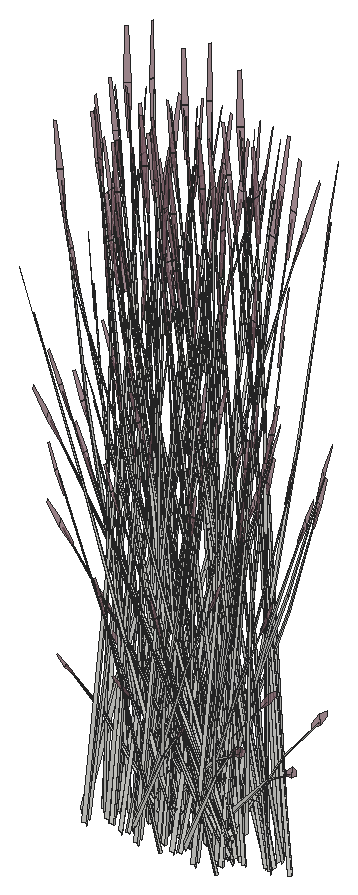
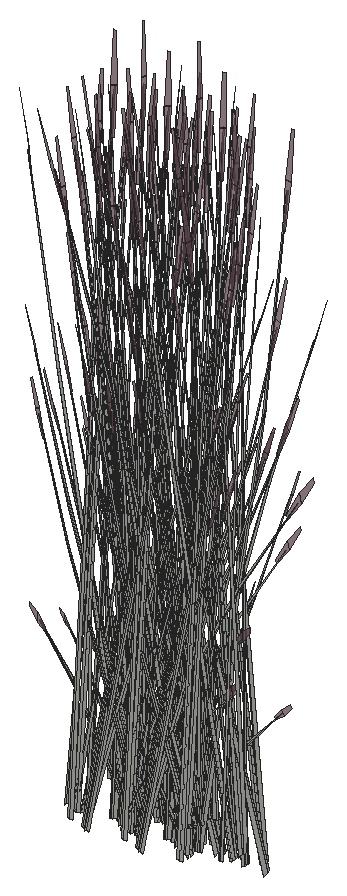
# SketchUp Ruby script. Lengths in inches.
U = 1.inch
M = Sketchup.active_model
def pt(a) = Geom::Point3d.new(a.map { |v| v * U })
def face(e, loops, mat)
  f = e.add_face(loops[0].map { |a| pt(a) })
  loops[1..].each { |l| e.add_face(l.map { |a| pt(a) }).erase! }
  f.material = f.back_material = mat if mat
  f
end
# faces: each face lists its corners as indices into pts; further lists are holes
def faces(e, pts, list, mat = nil) = list.each { |f| face(e, (f[0].is_a?(Array) ? f : [f]).map { |l| l.map { |i| pts[i] } }, mat) }
# xy, xz, yz: faces in a plane at the given z, y or x. An outline is a flat list of corners, or four numbers for a rectangle; further outlines are holes
def ring(l) = l.size == 4 ? [[l[0], l[1]], [l[2], l[1]], [l[2], l[3]], [l[0], l[3]]] : l.each_slice(2).to_a
def flat(e, list, mat, &to3) = list.each { |f| face(e, (f[0].is_a?(Array) ? f : [f]).map { |l| ring(l).map { |u, v| to3.(u, v) } }, mat) }
def xy(e, z, list, mat = nil) = flat(e, list, mat) { |x, y| [x, y, z] }
def xz(e, y, list, mat = nil) = flat(e, list, mat) { |x, z| [x, y, z] }
def yz(e, x, list, mat = nil) = flat(e, list, mat) { |y, z| [x, y, z] }
def lines(e, pts, list) = list.each { |a, b| e.add_line(pt(pts[a]), pt(pts[b])) }
# prism: a flat outline (further loops are holes) pulled along v
def prism(e, loops, v, mat = nil)
  f = face(e, loops, mat); d = Geom::Vector3d.new(v.map { |x| x * U })
  f.pushpull(f.normal.samedirection?(d) ? d.length : -d.length)
end
def box(e, o, s, mat = nil) = prism(e, [[o, [o[0] + s[0], o[1], o[2]], [o[0] + s[0], o[1] + s[1], o[2]], [o[0], o[1] + s[1], o[2]]]], [0, 0, s[2]], mat)
def at(x, y, z, deg = 0) = Geom::Transformation.translation(pt([x, y, z])) * Geom::Transformation.rotation(ORIGIN, Z_AXIS, deg.degrees)
def axes(o, x, y, z) = Geom::Transformation.new([*x, 0, *y, 0, *z, 0, *pt(o).to_a, 1])
def part(name) = M.definitions.add(name)
# library, detail: a bought-in or finely detailed component or shape, given as its bounding box
def library(name, o, s) = part(name).tap { |d| box(d.entities, o, s) }
def detail(e, o, s) = box(e.add_group.entities, o, s)
def put(e, d, t, mat = nil) = e.add_instance(d, t).tap { |i| i.material = mat if mat }
def group(e, t, mat = nil) = e.add_group.tap { |g| g.transformation = t; g.material = mat if mat }.entities
root = M.entities
M.materials.add("LightPink_Translucent").color = [144, 107, 117]
M.materials["LightPink_Translucent"].alpha = 0.75
c1 = part("blade")
p = [[2.15,0.21,22],[0,0.17,0],[0.09,0.45,0],[2.18,0.31,22],[2.29,0.31,22],[0.38,0.45,0],
  [2.48,0.24,33],[2.49,0.24,33],[2.48,0.22,33]]
faces(c1.entities,p,[[0,1,2,3],[4,5,2,3],[6,3,4,7],[8,0,3,6]])
c2 = part("seeds")
p = [[0.3,-0.1,1.38],[-0.01,-0.03,1.59],[-0.01,-0.03,0.03],[0.14,-0.07,-0.07],[0.29,-0.03,3],[0.15,0.01,3.11]]
faces(c2.entities,p,[[0,1,2,3],[1,0,4,5]],"LightPink_Translucent")
c3 = part("blade with seeds")
put(c3.entities,c1,at(0,0,0))
put(c3.entities,c2,axes([2.4,0.25,30.99],[1.5799,-0.05474,1.17369],[-0.12525,1.92788,0.29478],[-0.07173,-0.02425,1.56792]))
put(root,c3,axes([667.22,337.86,391.67],[0.60889,-0.28548,-0.4121],[0.36394,0.51192,0],[0.13868,-0.06502,1.30728]))
put(root,c3,axes([670.97,337.86,391.67],[0.60889,-0.28548,-0.4121],[0.36394,0.51192,0],[0.13868,-0.06502,1.30728]))
put(root,c3,axes([675.15,337.86,391.67],[0.60889,-0.28548,-0.4121],[0.36394,0.51192,0],[0.13868,-0.06502,1.30728]))
put(root,c3,axes([670.83,338.85,392.15],[-0.23242,-0.01691,1.18691],[-0.23811,-0.45367,-0.25526],[0.28553,-0.12834,0.50747]))
put(root,c3,axes([674.58,338.85,392.15],[-0.23242,-0.01691,1.18691],[-0.23811,-0.45367,-0.25526],[0.28553,-0.12834,0.50747]))
put(root,c3,axes([673.16,338.33,394.23],[0.53728,-0.42137,0.44623],[0.46337,0.44748,0.36794],[-0.25207,-0.07773,0.92337]))
put(root,c3,axes([677.23,338.33,394.23],[0.53728,-0.42137,0.44623],[0.46337,0.44748,0.36794],[-0.25207,-0.07773,0.92337]))
put(root,c3,axes([672.1,339.29,393.91],[-0.08498,-0.00434,1.47228],[-0.35287,-0.46464,-0.13912],[0.14171,-0.15278,0.26054]))
put(root,c3,axes([675.85,339.29,393.91],[-0.08498,-0.00434,1.47228],[-0.35287,-0.46464,-0.13912],[0.14171,-0.15278,0.26054]))
put(root,c3,axes([667.94,339.03,391.71],[0.43821,-0.42916,-0.51753],[0.54436,0.38915,-0.13583],[0.1756,-0.10706,1.14236]))
put(root,c3,axes([671.69,339.03,391.71],[0.43821,-0.42916,-0.51753],[0.54436,0.38915,-0.13583],[0.1756,-0.10706,1.14236]))
put(root,c3,axes([675.87,339.03,391.71],[0.43821,-0.42916,-0.51753],[0.54436,0.38915,-0.13583],[0.1756,-0.10706,1.14236]))
put(root,c3,axes([671.1,338.02,392.3],[-0.2167,0.29065,0.95334],[-0.18626,-0.3905,0.70045],[0.17898,-0.09785,0.20998]))
put(root,c3,axes([674.85,338.02,392.3],[-0.2167,0.29065,0.95334],[-0.18626,-0.3905,0.70045],[0.17898,-0.09785,0.20998]))
put(root,c3,axes([670.79,339.11,393.76],[0.56631,-0.0816,-0.29394],[0.14954,0.46647,0.37948],[0.16229,-0.12529,0.72609]))
put(root,c3,axes([674.54,339.11,393.76],[0.56631,-0.0816,-0.29394],[0.14954,0.46647,0.37948],[0.16229,-0.12529,0.72609]))
put(root,c3,axes([673.41,338.33,393.93],[0.03276,-0.43418,0.05337],[0.49468,0.0119,0.42015],[-0.18949,-0.04543,0.64067]))
put(root,c3,axes([677.48,338.33,393.93],[0.03276,-0.43418,0.05337],[0.49468,0.0119,0.42015],[-0.18949,-0.04543,0.64067]))
put(root,c3,axes([670.93,339.79,391.83],[0.31565,-0.51449,-0.37133],[0.65588,0.24761,0.17871],[0,-0.1186,1.19224]))
put(root,c3,axes([675.11,339.79,391.83],[0.31565,-0.51449,-0.37133],[0.65588,0.24761,0.17871],[0,-0.1186,1.19224]))
put(root,c3,axes([679.18,339.79,391.83],[0.31565,-0.51449,-0.37133],[0.65588,0.24761,0.17871],[0,-0.1186,1.19224]))
put(root,c3,axes([677.29,338.47,393.76],[-0.37017,-0.35748,-0.29394],[0.42268,-0.3384,0.37948],[-0.21476,-0.05149,0.72609]))
put(root,c3,axes([667.47,339.53,392.21],[-0.07581,-0.65151,-0.24149],[0.7896,-0.03939,-0.41502],[0.13904,-0.08678,1.32557]))
put(root,c3,axes([671.22,339.53,392.21],[-0.07581,-0.65151,-0.24149],[0.7896,-0.03939,-0.41502],[0.13904,-0.08678,1.32557]))
put(root,c3,axes([675.4,339.53,392.21],[-0.07581,-0.65151,-0.24149],[0.7896,-0.03939,-0.41502],[0.13904,-0.08678,1.32557]))
put(root,c3,axes([669.26,339.57,391.68],[0.45414,-0.35624,-0.25712],[0.45414,0.35624,0.25712],[0,-0.11474,1.15348]))
put(root,c3,axes([673.44,339.57,391.68],[0.45414,-0.35624,-0.25712],[0.45414,0.35624,0.25712],[0,-0.11474,1.15348]))
put(root,c3,axes([677.51,339.57,391.68],[0.45414,-0.35624,-0.25712],[0.45414,0.35624,0.25712],[0,-0.11474,1.15348]))
put(root,c3,axes([673.26,337.86,391.77],[-0.18768,0.46622,-0.03231],[-0.57763,-0.14342,-0.14649],[-0.0877,-0.07626,0.48318]))
put(root,c3,axes([677.33,337.86,391.77],[-0.18768,0.46622,-0.03231],[-0.57763,-0.14342,-0.14649],[-0.0877,-0.07626,0.48318]))
put(root,c3,axes([670.33,339.38,394.19],[-0.56631,0.0816,0.29394],[-0.14954,-0.46647,-0.37948],[0.16229,-0.12529,0.72609]))
put(root,c3,axes([674.08,339.38,394.19],[-0.56631,0.0816,0.29394],[-0.14954,-0.46647,-0.37948],[0.16229,-0.12529,0.72609]))
put(root,c3,axes([678.26,339.38,394.19],[-0.56631,0.0816,0.29394],[-0.14954,-0.46647,-0.37948],[0.16229,-0.12529,0.72609]))
put(root,c3,axes([670.85,340.21,392.21],[-0.73268,-0.27244,-0.24149],[0.35279,-0.57501,-0.41502],[-0.02303,-0.14118,1.32557]))
put(root,c3,axes([675.03,340.21,392.21],[-0.73268,-0.27244,-0.24149],[0.35279,-0.57501,-0.41502],[-0.02303,-0.14118,1.32557]))
put(root,c3,axes([679.1,340.21,392.21],[-0.73268,-0.27244,-0.24149],[0.35279,-0.57501,-0.41502],[-0.02303,-0.14118,1.32557]))
put(root,c3,axes([672.95,339.99,391.97],[-0.81352,0,0],[0,-0.63814,-0.42834],[0,-0.14534,1.3588]))
put(root,c3,axes([677.02,339.99,391.97],[-0.81352,0,0],[0,-0.63814,-0.42834],[0,-0.14534,1.3588]))
put(root,c3,axes([677.15,338.85,392.15],[0.12702,0.15896,1.18691],[-0.2927,0.4321,-0.25526],[-0.30054,-0.10328,0.50747]))
put(root,c3,axes([667.36,338.09,391.68],[0.60696,0.14127,-0.25712],[-0.15283,0.49751,0.25712],[0.12236,-0.05737,1.15348]))
put(root,c3,axes([671.11,338.09,391.68],[0.60696,0.14127,-0.25712],[-0.15283,0.49751,0.25712],[0.12236,-0.05737,1.15348]))
put(root,c3,axes([675.29,338.09,391.68],[0.60696,0.14127,-0.25712],[-0.15283,0.49751,0.25712],[0.12236,-0.05737,1.15348]))
put(root,c3,axes([677.68,338.71,394.13],[-0.65035,-0.01375,-0.58968],[0.04368,-0.5789,0.07116],[-0.27552,-0.06109,0.83415]))
put(root,c3,axes([670.84,339.31,393.93],[0.44663,0.24013,0.05337],[-0.26003,0.34195,0.42015],[0.14319,-0.11055,0.64067]))
put(root,c3,axes([674.59,339.31,393.93],[0.44663,0.24013,0.05337],[-0.26003,0.34195,0.42015],[0.14319,-0.11055,0.64067]))
put(root,c3,axes([670.72,339.21,393.93],[0.16135,0.52549,0.39842],[-0.63294,0.0912,0.32852],[0.18654,-0.12359,0.82444]))
put(root,c3,axes([674.47,339.21,393.93],[0.16135,0.52549,0.39842],[-0.63294,0.0912,0.32852],[0.18654,-0.12359,0.82444]))
put(root,c3,axes([672.42,339.84,393.91],[0.09028,-0.08697,1.45204],[-0.11555,-0.53348,-0.22964],[0.22652,-0.10115,0.11645]))
put(root,c3,axes([676.17,339.84,393.91],[0.09028,-0.08697,1.45204],[-0.11555,-0.53348,-0.22964],[0.22652,-0.10115,0.11645]))
put(root,c3,axes([673.58,339.82,391.93],[-0.60515,0.48003,0.25528],[-0.60552,-0.47498,-0.30288],[-0.02113,-0.13632,1.36855]))
put(root,c3,axes([677.65,339.82,391.93],[-0.60515,0.48003,0.25528],[-0.60552,-0.47498,-0.30288],[-0.02113,-0.13632,1.36855]))
put(root,c3,axes([676.8,337.76,393.91],[0.04823,0.05698,1.47228],[-0.23252,0.51221,-0.13912],[-0.23548,0.00371,0.26054]))
put(root,c3,axes([671.32,340.04,392.02],[0.73304,0.27674,0.19974],[-0.35279,0.57501,0.41502],[0,-0.13255,1.3325]))
put(root,c3,axes([675.5,340.04,392.02],[0.73304,0.27674,0.19974],[-0.35279,0.57501,0.41502],[0,-0.13255,1.3325]))
put(root,c3,axes([675.22,340.82,392.02],[0.17244,-0.67657,-0.19446],[0.81759,0.11793,0.42555],[-0.14286,-0.09343,1.29846]))
put(root,c3,axes([679.28,340.82,392.02],[0.17244,-0.67657,-0.19446],[0.81759,0.11793,0.42555],[-0.14286,-0.09343,1.29846]))
put(root,c3,axes([677.46,338.82,393.89],[-0.47241,0.37822,-0.42412],[-0.41372,-0.39954,-0.32852],[-0.24002,-0.05755,0.81151]))
put(root,c3,axes([673.74,338.65,394.19],[0.37017,0.35748,0.29394],[-0.42268,0.3384,-0.37948],[-0.21476,-0.05149,0.72609]))
put(root,c3,axes([677.8125,338.65,394.19],[0.37017,0.35748,0.29394],[-0.42268,0.3384,-0.37948],[-0.21476,-0.05149,0.72609]))
put(root,c3,axes([672.33,339.32,392.3],[0.41536,-0.04086,0.95334],[-0.26347,0.35999,0.70045],[-0.20525,-0.054,0.20998]))
put(root,c3,axes([676.4,339.32,392.3],[0.41536,-0.04086,0.95334],[-0.26347,0.35999,0.70045],[-0.20525,-0.054,0.20998]))
put(root,c3,axes([671.08,339.66,392.26],[-0.70648,0.03525,0.37133],[-0.06389,-0.58508,-0.17871],[0.12647,-0.0593,1.19224]))
put(root,c3,axes([675.26,339.66,392.26],[-0.70648,0.03525,0.37133],[-0.06389,-0.58508,-0.17871],[0.12647,-0.0593,1.19224]))
put(root,c3,axes([677.71,338.43,394.18],[-0.03484,0.58066,-0.10093],[-0.65957,-0.01587,-0.56021],[-0.25402,-0.04034,0.85122]))
put(root,c3,axes([669.26,340.08,392.06],[0,0.57097,0.4121],[-0.72788,0,0],[0,-0.13004,1.30728]))
put(root,c3,axes([673.44,340.08,392.06],[0,0.57097,0.4121],[-0.72788,0,0],[0,-0.13004,1.30728]))
put(root,c3,axes([677.51,340.08,392.06],[0,0.57097,0.4121],[-0.72788,0,0],[0,-0.13004,1.30728]))
put(root,c3,axes([670.65,340.65,394.18],[-0.32734,-0.51701,-0.10093],[0.58097,-0.25407,-0.56021],[0.24483,-0.06821,0.85122]))
put(root,c3,axes([674.4,340.65,394.18],[-0.32734,-0.51701,-0.10093],[0.58097,-0.25407,-0.56021],[0.24483,-0.06821,0.85122]))
put(root,c3,axes([670.62,340.21,393.89],[0.17625,-0.51936,-0.42412],[0.60429,0.17802,-0.32852],[0.2433,-0.04762,0.81151]))
put(root,c3,axes([674.37,340.21,393.89],[0.17625,-0.51936,-0.42412],[0.60429,0.17802,-0.32852],[0.2433,-0.04762,0.81151]))
put(root,c3,axes([669.66,338.1,391.97],[0.40676,-0.57214,0],[0.68052,0.31907,-0.42834],[0.15499,0.07267,1.3588]))
put(root,c3,axes([673.41,338.1,391.97],[0.40676,-0.57214,0],[0.68052,0.31907,-0.42834],[0.15499,0.07267,1.3588]))
put(root,c3,axes([676.87,339.23,393.22],[0.26985,-0.01293,1.42242],[-0.17902,0.56047,0.11501],[-0.38456,-0.03467,0.60807]))
put(root,c3,axes([675.16,340.54,391.83],[-0.39083,-0.47924,-0.37133],[0.59199,-0.33747,0.17871],[-0.12647,-0.0593,1.19224]))
put(root,c3,axes([679.23,340.54,391.83],[-0.39083,-0.47924,-0.37133],[0.59199,-0.33747,0.17871],[-0.12647,-0.0593,1.19224]))
put(root,c3,axes([671.06,339.87,391.96],[0.28286,0.63846,0.37976],[-0.80821,0.22202,0.14902],[0.00988,-0.11732,1.31851]))
put(root,c3,axes([675.24,339.87,391.96],[0.28286,0.63846,0.37976],[-0.80821,0.22202,0.14902],[0.00988,-0.11732,1.31851]))
put(root,c3,axes([679.31,339.87,391.96],[0.28286,0.63846,0.37976],[-0.80821,0.22202,0.14902],[0.00988,-0.11732,1.31851]))
put(root,c3,axes([671.26,340.36,391.65],[-0.41902,0.06852,1.17514],[-0.0667,-0.54541,0.06726],[0.29348,-0.08255,0.6687]))
put(root,c3,axes([675.01,340.36,391.65],[-0.41902,0.06852,1.17514],[-0.0667,-0.54541,0.06726],[0.29348,-0.08255,0.6687]))
put(root,c3,axes([672.03,339.875,391.875],[-0.40335,-0.3651,-0.05385],[0.44175,-0.33453,-0.24415],[0.12517,-0.02355,0.8053]))
put(root,c3,axes([675.78,339.875,391.875],[-0.40335,-0.3651,-0.05385],[0.44175,-0.33453,-0.24415],[0.12517,-0.02355,0.8053]))
put(root,c3,axes([670.92,340.37,392.26],[-0.31565,0.51449,0.37133],[-0.65588,-0.24761,-0.17871],[0,-0.1186,1.19224]))
put(root,c3,axes([675.1,340.37,392.26],[-0.31565,0.51449,0.37133],[-0.65588,-0.24761,-0.17871],[0,-0.1186,1.19224]))
put(root,c3,axes([679.17,340.37,392.26],[-0.31565,0.51449,0.37133],[-0.65588,-0.24761,-0.17871],[0,-0.1186,1.19224]))
put(root,c3,axes([672.07,339.92,391.83],[0,-0.66065,0],[0.81352,0,0],[0,0,1.48949]))
put(root,c3,axes([676.26,339.92,391.83],[0,-0.66065,0],[0.81352,0,0],[0,0,1.48949]))
put(root,c3,axes([669.3125,338.39,392.06],[-0.60889,-0.28548,0.4121],[0.36394,-0.51192,0],[0.13868,0.06502,1.30728]))
put(root,c3,axes([673.0625,338.39,392.06],[-0.60889,-0.28548,0.4121],[0.36394,-0.51192,0],[0.13868,0.06502,1.30728]))
put(root,c3,axes([677.24,338.39,392.06],[-0.60889,-0.28548,0.4121],[0.36394,-0.51192,0],[0.13868,0.06502,1.30728]))
put(root,c3,axes([670.5,340.4,394.13],[0.57168,-0.25217,-0.58968],[0.3186,0.51908,0.07116],[0.27622,-0.05897,0.83415]))
put(root,c3,axes([674.25,340.4,394.13],[0.57168,-0.25217,-0.58968],[0.3186,0.51908,0.07116],[0.27622,-0.05897,0.83415]))
put(root,c3,axes([674.81,340.73,391.71],[-0.67676,-0.09361,-0.51753],[0.14281,-0.57742,-0.13583],[-0.20196,-0.06997,1.14236]))
put(root,c3,axes([678.875,340.73,391.71],[-0.67676,-0.09361,-0.51753],[0.14281,-0.57742,-0.13583],[-0.20196,-0.06997,1.14236]))
put(root,c3,axes([667.94,339.51,391.96],[-0.53943,0.51816,0.37976],[-0.64086,-0.4574,0.14902],[0.13005,-0.05171,1.31851]))
put(root,c3,axes([671.6875,339.51,391.96],[-0.53943,0.51816,0.37976],[-0.64086,-0.4574,0.14902],[0.13005,-0.05171,1.31851]))
put(root,c3,axes([675.87,339.51,391.96],[-0.53943,0.51816,0.37976],[-0.64086,-0.4574,0.14902],[0.13005,-0.05171,1.31851]))
put(root,c3,axes([672.28,340.43,391.91],[-0.60515,-0.49144,-0.05089],[0.60552,-0.49174,0],[-0.02113,-0.01716,1.45724]))
put(root,c3,axes([676.46,340.43,391.91],[-0.60515,-0.49144,-0.05089],[0.60552,-0.49174,0],[-0.02113,-0.01716,1.45724]))
put(root,c3,axes([680.53,340.43,391.91],[-0.60515,-0.49144,-0.05089],[0.60552,-0.49174,0],[-0.02113,-0.01716,1.45724]))
put(root,c3,axes([670.75,338.65,392.05],[-0.18794,0.56744,0.14643],[-0.68774,-0.16058,0.29122],[0.1188,-0.00276,1.33138]))
put(root,c3,axes([674.93,338.65,392.05],[-0.18794,0.56744,0.14643],[-0.68774,-0.16058,0.29122],[0.1188,-0.00276,1.33138]))
put(root,c3,axes([670.42,340.5,394.19],[-0.54068,-0.15928,0.29394],[0.1577,-0.46469,-0.37948],[0.21769,-0.04261,0.72609]))
put(root,c3,axes([674.17,340.5,394.19],[-0.54068,-0.15928,0.29394],[0.1577,-0.46469,-0.37948],[0.21769,-0.04261,0.72609]))
put(root,c3,axes([676.76,339.65,393.93],[0.18381,-0.5206,0.39842],[0.60429,0.17802,0.32852],[-0.23764,0.03129,0.82444]))
put(root,c3,axes([666.72,339.11,391.32],[-0.64037,0.22859,1.07011],[-0.20382,-0.65589,0.4158],[0.39323,0.01091,1.21713]))
put(root,c3,axes([670.47,339.11,391.32],[-0.64037,0.22859,1.07011],[-0.20382,-0.65589,0.4158],[0.39323,0.01091,1.21713]))
put(root,c3,axes([668.44,339.28,392.17],[0.12551,-0.50956,0.12018],[0.6132,0.08845,-0.34318],[0.1116,0.05232,1.05198]))
put(root,c3,axes([672.1875,339.28,392.17],[0.12551,-0.50956,0.12018],[0.6132,0.08845,-0.34318],[0.1116,0.05232,1.05198]))
put(root,c3,axes([676.37,339.28,392.17],[0.12551,-0.50956,0.12018],[0.6132,0.08845,-0.34318],[0.1116,0.05232,1.05198]))
put(root,c3,axes([676.71,339.51,393.93],[-0.23895,-0.38931,0.05337],[0.43573,-0.19055,0.42015],[-0.19208,0.0376,0.64067]))
put(root,c3,axes([671.13,340.49,391.96],[0.82229,0.1203,0.37976],[-0.16734,0.67942,0.14902],[-0.12017,-0.06561,1.31851]))
put(root,c3,axes([675.31,340.49,391.96],[0.82229,0.1203,0.37976],[-0.16734,0.67942,0.14902],[-0.12017,-0.06561,1.31851]))
put(root,c3,axes([679.38,340.49,391.96],[0.82229,0.1203,0.37976],[-0.16734,0.67942,0.14902],[-0.12017,-0.06561,1.31851]))
put(root,c3,axes([671.72,340,391.24],[-0.034,-0.08668,1.46364],[0.23582,-0.50706,-0.2236],[0.23788,-0.00729,0.24931]))
put(root,c3,axes([675.47,340,391.24],[-0.034,-0.08668,1.46364],[0.23582,-0.50706,-0.2236],[0.23788,-0.00729,0.24931]))
put(root,c3,axes([676.7,339.91,391.24],[0.0165,0.08998,1.46364],[-0.33262,0.46992,-0.2236],[-0.23626,-0.02369,0.24931]))
put(root,c3,axes([668.18,339.42,392.26],[-0.39083,-0.47924,0.37133],[0.59199,-0.33747,-0.17871],[0.12647,0.0593,1.19224]))
put(root,c3,axes([671.93,339.42,392.26],[-0.39083,-0.47924,0.37133],[0.59199,-0.33747,-0.17871],[0.12647,0.0593,1.19224]))
put(root,c3,axes([676.11,339.42,392.26],[-0.39083,-0.47924,0.37133],[0.59199,-0.33747,-0.17871],[0.12647,0.0593,1.19224]))
put(root,c3,axes([674.09,341.61,391.68],[-0.15283,-0.49751,-0.25712],[0.60696,-0.14127,0.25712],[-0.12236,-0.05737,1.15348]))
put(root,c3,axes([678.16,341.61,391.68],[-0.15283,-0.49751,-0.25712],[0.60696,-0.14127,0.25712],[-0.12236,-0.05737,1.15348]))
put(root,c3,axes([670.6875,341.58,392.05],[0.6991,-0.15154,0.14643],[0.17263,0.56398,0.29122],[-0.06235,-0.08217,1.33138]))
put(root,c3,axes([674.87,341.58,392.05],[0.6991,-0.15154,0.14643],[0.17263,0.56398,0.29122],[-0.06235,-0.08217,1.33138]))
put(root,c3,axes([678.9375,341.58,392.05],[0.6991,-0.15154,0.14643],[0.17263,0.56398,0.29122],[-0.06235,-0.08217,1.33138]))
put(root,c3,axes([668.38,339.45,392.21],[0.65687,-0.37907,-0.24149],[0.43681,0.53562,-0.41502],[0.16207,0.0544,1.32557]))
put(root,c3,axes([672.125,339.45,392.21],[0.65687,-0.37907,-0.24149],[0.43681,0.53562,-0.41502],[0.16207,0.0544,1.32557]))
put(root,c3,axes([676.31,339.45,392.21],[0.65687,-0.37907,-0.24149],[0.43681,0.53562,-0.41502],[0.16207,0.0544,1.32557]))
put(root,c3,axes([670.99,340.45,393.76],[0.54068,0.15928,-0.29394],[-0.1577,0.46469,0.37948],[0.21769,-0.04261,0.72609]))
put(root,c3,axes([674.74,340.45,393.76],[0.54068,0.15928,-0.29394],[-0.1577,0.46469,0.37948],[0.21769,-0.04261,0.72609]))
put(root,c3,axes([673.92,341.82,391.67],[-0.60889,-0.28548,-0.4121],[0.36394,-0.51192,0],[-0.13868,-0.06502,1.30728]))
put(root,c3,axes([677.99,341.82,391.67],[-0.60889,-0.28548,-0.4121],[0.36394,-0.51192,0],[-0.13868,-0.06502,1.30728]))
put(root,c3,axes([670.03,338.44,391.67],[0.60889,0.28548,-0.4121],[-0.36394,0.51192,0],[0.13868,0.06502,1.30728]))
put(root,c3,axes([673.78,338.44,391.67],[0.60889,0.28548,-0.4121],[-0.36394,0.51192,0],[0.13868,0.06502,1.30728]))
put(root,c3,axes([676.63,339.71,393.76],[-0.54068,-0.15928,-0.29394],[0.1577,-0.46469,0.37948],[-0.21769,0.04261,0.72609]))
